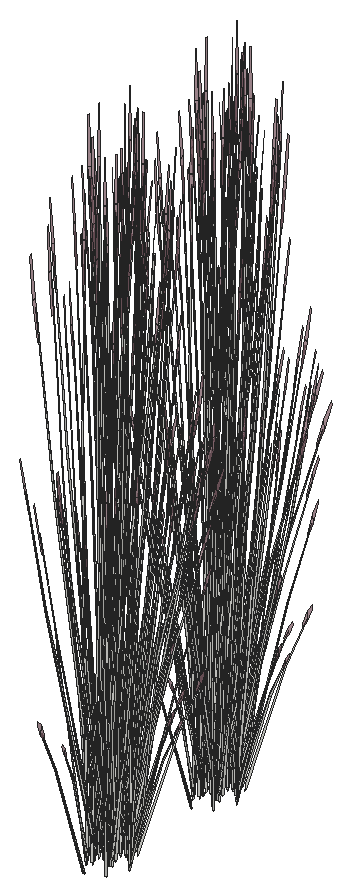
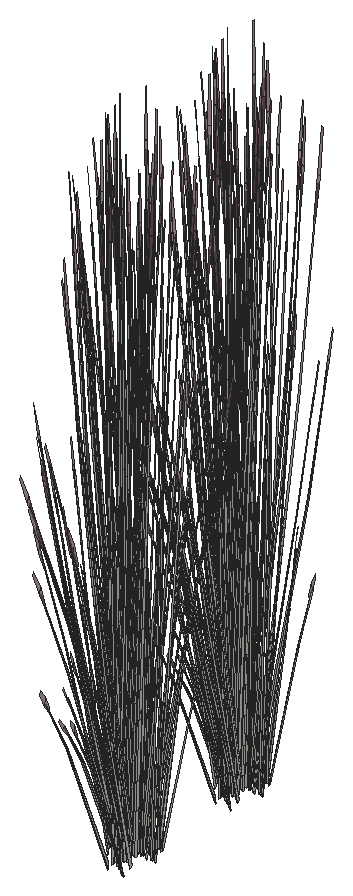
# SketchUp Ruby script. Lengths in inches.
U = 1.inch
M = Sketchup.active_model
def pt(a) = Geom::Point3d.new(a.map { |v| v * U })
def face(e, loops, mat)
  f = e.add_face(loops[0].map { |a| pt(a) })
  loops[1..].each { |l| e.add_face(l.map { |a| pt(a) }).erase! }
  f.material = f.back_material = mat if mat
  f
end
# faces: each face lists its corners as indices into pts; further lists are holes
def faces(e, pts, list, mat = nil) = list.each { |f| face(e, (f[0].is_a?(Array) ? f : [f]).map { |l| l.map { |i| pts[i] } }, mat) }
# xy, xz, yz: faces in a plane at the given z, y or x. An outline is a flat list of corners, or four numbers for a rectangle; further outlines are holes
def ring(l) = l.size == 4 ? [[l[0], l[1]], [l[2], l[1]], [l[2], l[3]], [l[0], l[3]]] : l.each_slice(2).to_a
def flat(e, list, mat, &to3) = list.each { |f| face(e, (f[0].is_a?(Array) ? f : [f]).map { |l| ring(l).map { |u, v| to3.(u, v) } }, mat) }
def xy(e, z, list, mat = nil) = flat(e, list, mat) { |x, y| [x, y, z] }
def xz(e, y, list, mat = nil) = flat(e, list, mat) { |x, z| [x, y, z] }
def yz(e, x, list, mat = nil) = flat(e, list, mat) { |y, z| [x, y, z] }
def lines(e, pts, list) = list.each { |a, b| e.add_line(pt(pts[a]), pt(pts[b])) }
# prism: a flat outline (further loops are holes) pulled along v
def prism(e, loops, v, mat = nil)
  f = face(e, loops, mat); d = Geom::Vector3d.new(v.map { |x| x * U })
  f.pushpull(f.normal.samedirection?(d) ? d.length : -d.length)
end
def box(e, o, s, mat = nil) = prism(e, [[o, [o[0] + s[0], o[1], o[2]], [o[0] + s[0], o[1] + s[1], o[2]], [o[0], o[1] + s[1], o[2]]]], [0, 0, s[2]], mat)
def at(x, y, z, deg = 0) = Geom::Transformation.translation(pt([x, y, z])) * Geom::Transformation.rotation(ORIGIN, Z_AXIS, deg.degrees)
def axes(o, x, y, z) = Geom::Transformation.new([*x, 0, *y, 0, *z, 0, *pt(o).to_a, 1])
def part(name) = M.definitions.add(name)
# library, detail: a bought-in or finely detailed component or shape, given as its bounding box
def library(name, o, s) = part(name).tap { |d| box(d.entities, o, s) }
def detail(e, o, s) = box(e.add_group.entities, o, s)
def put(e, d, t, mat = nil) = e.add_instance(d, t).tap { |i| i.material = mat if mat }
def group(e, t, mat = nil) = e.add_group.tap { |g| g.transformation = t; g.material = mat if mat }.entities
root = M.entities
M.materials.add("LightPink_Translucent").color = [144, 107, 117]
M.materials["LightPink_Translucent"].alpha = 0.75
c1 = part("blade")
p = [[2.15,0.21,22],[0,0.17,0],[0.09,0.45,0],[2.18,0.31,22],[2.29,0.31,22],[0.38,0.45,0],
  [2.48,0.24,33],[2.49,0.24,33],[2.48,0.22,33]]
faces(c1.entities,p,[[0,1,2,3],[4,5,2,3],[6,3,4,7],[8,0,3,6]])
c2 = part("seeds")
p = [[0.3,-0.1,1.38],[-0.01,-0.03,1.59],[-0.01,-0.03,0.03],[0.14,-0.07,-0.07],[0.29,-0.03,3],[0.15,0.01,3.11]]
faces(c2.entities,p,[[0,1,2,3],[1,0,4,5]],"LightPink_Translucent")
c3 = part("blade with seeds")
put(c3.entities,c1,at(0,0,0))
put(c3.entities,c2,axes([2.4,0.25,30.99],[1.5799,-0.05474,1.17369],[-0.12525,1.92788,0.29478],[-0.07173,-0.02425,1.56792]))
put(root,c3,axes([401.98,775.3,1.49],[-0.0592,0.0168,1.76342],[-0.32738,-0.18913,-0.26939],[0.00549,-0.15776,0.30037]))
put(root,c3,axes([402.97,776.51,4.98],[0.00918,-0.43138,-0.71045],[0.38672,0.02897,0.08574],[0.04081,-0.18275,1.00501]))
put(root,c3,axes([402.3,775.82,4.53],[0.1064,-0.35863,-0.35414],[0.31043,0.1046,0.4572],[-0.02846,-0.14439,0.87481]))
put(root,c3,axes([402.53,776.3,3.875],[-0.06572,0.16029,1.71376],[-0.27569,-0.33172,0.13857],[0.12437,-0.20675,0.73262]))
put(root,c3,axes([402.14,776.07,4.68],[-0.34695,-0.11691,-0.51099],[0.11892,-0.40083,-0.3958],[-0.03181,-0.16138,0.97773]))
put(root,c3,axes([402.35,775.0625,2.77],[0.04528,0.27194,1.1486],[-0.25117,-0.15062,0.84392],[0.02703,-0.13924,0.25299]))
put(root,c3,axes([402.89,776.37,4.68],[-0.25266,-0.31335,-0.51099],[0.2669,-0.27442,-0.3958],[0.03844,-0.15921,0.97773]))
put(root,c3,axes([403.13,776.26,4.53],[0.23881,-0.24554,-0.35414],[0.22606,0.28036,0.4572],[0.0344,-0.14245,0.87481]))
put(root,c3,axes([401.49,777.57,2.1],[-0.14494,-0.47823,-0.69835],[0.41752,-0.17223,-0.18329],[-0.01602,-0.16194,1.54149]))
put(root,c3,axes([403.43,776.11,1.49],[-0.05283,-0.03674,1.76342],[-0.13569,-0.41045,-0.26939],[0.09154,-0.11138,0.30037]))
put(root,c3,axes([403.42,777.26,4.98],[0.18436,-0.36797,-0.71045],[0.32306,0.26151,0.08574],[0.11008,-0.13332,1.00501]))
put(root,c3,axes([401.43,776.19,2.375],[-0.22066,-0.46731,0],[0.36918,-0.26061,-0.51607],[0.08408,-0.05936,1.63711]))
put(root,c3,axes([403.41,777.09,4.68],[-0.09067,-0.42583,-0.51099],[0.34336,-0.07449,-0.3958],[0.0984,-0.11438,0.97773]))
put(root,c3,axes([401.92,775.63,2.13],[-0.2439,0.26754,-0.03893],[-0.22348,-0.29302,-0.17649],[-0.01573,-0.08303,0.58215]))
put(root,c3,axes([400.63,777.5,2.02],[0,-0.46636,-0.49651],[0.39487,0,0],[0,-0.10622,1.57504]))
put(root,c3,axes([401.73,776.12,2.02],[0.33032,-0.23318,-0.49651],[0.19744,0.41812,0],[0.07523,-0.05311,1.57504]))
put(root,c3,axes([403.69,776.93,2.59],[-0.12609,-0.01381,1.43002],[-0.12917,-0.37055,-0.30754],[0.1549,-0.10482,0.61141]))
put(root,c3,axes([402.12,777.08,2.06],[0.23773,-0.35053,-0.62353],[0.29532,0.31785,-0.16365],[0.09526,-0.08744,1.37633]))
put(root,c3,axes([403.84,776.25,2.77],[-0.11756,0.2374,1.1486],[-0.10105,-0.31895,0.84392],[0.09709,-0.07992,0.25299]))
put(root,c3,axes([403.67,777.14,4.53],[0.30722,-0.06665,-0.35414],[0.08112,0.381,0.4572],[0.08804,-0.10234,0.87481]))
put(root,c3,axes([401.71,777.69,2.21],[0.17124,-0.42022,-0.44739],[0.35581,0.20224,0.21531],[0,-0.09687,1.43643]))
put(root,c3,axes([401.86,777.48,2.67],[-0.04113,-0.53214,-0.29095],[0.42835,-0.03218,-0.50002],[0.07543,-0.07088,1.59708]))
put(root,c3,axes([400.8,777.51,2.03],[0.24637,-0.29097,-0.30978],[0.24637,0.29097,0.30978],[0,-0.09372,1.38974]))
put(root,c3,axes([401.67,778.04,2.67],[-0.39748,-0.22252,-0.29095],[0.19139,-0.46966,-0.50002],[-0.01249,-0.11531,1.59708]))
put(root,c3,axes([401.81,776.31,2.03],[0.32928,0.11539,-0.30978],[-0.08291,0.40636,0.30978],[0.06638,-0.04686,1.38974]))
put(root,c3,axes([401.92,777.9,2.43],[0.39767,0.22603,0.24065],[-0.19139,0.46966,0.50002],[0,-0.10827,1.60543]))
put(root,c3,axes([401.79,777.59,2.72],[-0.38326,0.02879,0.44739],[-0.03466,-0.47788,-0.21531],[0.06861,-0.04843,1.43643]))
put(root,c3,axes([400.8,777.93,2.48],[0,0.46636,0.49651],[-0.39487,0,0],[0,-0.10622,1.57504]))
put(root,c3,axes([403.57,778.04,4.68],[0.09562,-0.42421,-0.51099],[0.32782,0.1454,-0.3958],[0.13199,-0.0389,0.97773]))
put(root,c3,axes([403.06,776.3125,2.375],[0.22066,-0.46731,0],[0.36918,0.26061,-0.51607],[0.08408,0.05936,1.63711]))
put(root,c3,axes([401.78,777.76,2.36],[0.15345,0.52148,0.45755],[-0.43845,0.18134,0.17955],[0.00536,-0.09582,1.58856]))
put(root,c3,axes([403.92,778.16,1.98],[-0.22732,0.05597,1.41583],[-0.03618,-0.44548,0.08104],[0.15921,-0.06743,0.80566]))
put(root,c3,axes([404.34,777.76,2.26],[-0.21881,-0.29821,-0.06488],[0.23965,-0.27324,-0.29416],[0.0679,-0.01924,0.97024]))
put(root,c3,axes([401.7,778.17,2.72],[-0.17124,0.42022,0.44739],[-0.35581,-0.20224,-0.21531],[0,-0.09687,1.43643]))
put(root,c3,axes([402.33,777.8,2.21],[0,-0.53961,0],[0.44133,0,0],[0,0,1.79456]))
put(root,c3,axes([402.87,776.56,2.48],[-0.33032,-0.23318,0.49651],[0.19744,-0.41812,0],[0.07523,0.05311,1.57504]))
put(root,c3,axes([403.51,778.19,4.98],[0.31014,-0.20596,-0.71045],[0.17284,0.42397,0.08574],[0.14985,-0.04816,1.00501]))
put(root,c3,axes([402.12,777.46,2.36],[-0.29264,0.42323,0.45755],[-0.34767,-0.3736,0.17955],[0.07055,-0.04224,1.58856]))
put(root,c3,axes([402.44,778.22,2.3],[-0.32829,-0.4014,-0.06131],[0.32849,-0.40164,0],[-0.01146,-0.01402,1.75571]))
put(root,c3,axes([401.61,776.77,2.47],[-0.10196,0.46348,0.17642],[-0.3731,-0.13116,0.35086],[0.06445,-0.00226,1.60407]))
put(root,c3,axes([401.46,777.14,1.59],[-0.3474,0.18671,1.28929],[-0.11057,-0.53572,0.50096],[0.21332,0.00891,1.46642]))
put(root,c3,axes([402.39,777.28,2.62],[0.06809,-0.4162,0.1448],[0.33266,0.07225,-0.41347],[0.06054,0.04274,1.26744]))
put(root,c3,axes([401.82,778.27,2.36],[0.44609,0.09826,0.45755],[-0.09078,0.55493,0.17955],[-0.06519,-0.05359,1.58856]))
put(root,c3,axes([404.17,777.87,1.49],[-0.01845,-0.0708,1.76342],[0.12793,-0.41416,-0.26939],[0.12905,-0.00596,0.30037]))
put(root,c3,axes([402.25,777.39,2.72],[-0.21202,-0.39143,0.44739],[0.32115,-0.27564,-0.21531],[0.06861,0.04843,1.43643]))
put(root,c3,axes([401.58,779.16,2.47],[0.37926,-0.12378,0.17642],[0.09365,0.46065,0.35086],[-0.03382,-0.06712,1.60407]))
put(root,c3,axes([402.36,777.42,2.67],[0.35635,-0.30962,-0.29095],[0.23697,0.43749,-0.50002],[0.08792,0.04443,1.59708]))
put(root,c3,axes([403.78,778.23,4.53],[0.29332,0.1301,-0.35414],[-0.08555,0.37955,0.4572],[0.11809,-0.0348,0.87481]))
put(root,c3,axes([403.26,776.59,2.02],[0.33032,0.23318,-0.49651],[-0.19744,0.41812,0],[0.07523,0.05311,1.57504]))
put(root,c3,axes([402.63,777.92,2.21],[0.39487,0,0],[0,0.48281,0],[0,0,1.78407]))
put(root,c3,axes([402.74,776.79,2.47],[-0.37926,0.12378,0.17642],[-0.09365,-0.46065,0.35086],[0.03382,0.06712,1.60407]))
put(root,c3,axes([402.98,777.76,3.875],[-0.14639,0.01056,1.71376],[0.09712,-0.45778,0.13857],[0.20862,0.02831,0.73262]))
put(root,c3,axes([403.17,776.77,2.03],[0.08291,0.40636,-0.30978],[-0.32928,0.11539,0.30978],[0.06638,0.04686,1.38974]))
put(root,c3,axes([402.5,777.68,2.38],[-0.44609,-0.09826,0.49198],[0.09078,-0.55493,0.19306],[0.06519,0.05359,1.70813]))
put(root,c3,axes([402.15,779.05,2.2],[-0.11516,-0.40207,0],[0.32884,-0.1408,0],[0,0,1.54371]))
put(root,c3,axes([402.58,778.99,2.18],[0.37054,-0.15823,-0.19198],[0.1302,0.45581,0.00008],[0.0409,-0.01749,1.73897]))
put(root,c3,axes([402.71,779.18,2.47],[0.10196,-0.46348,0.17642],[0.3731,0.13116,0.35086],[-0.06445,0.00226,1.60407]))
put(root,c3,axes([402.62,778.13,2.21],[0.24637,0.30123,0],[-0.24637,0.30123,0],[0,0,1.69266]))
put(root,c3,axes([403.29,778,2.47],[-0.2773,-0.3397,0.17642],[0.27945,-0.32949,0.35086],[-0.03063,0.06937,1.60407]))
put(root,c3,axes([402.78,777.49,2.06],[0.36714,0.07646,-0.62353],[-0.07747,0.47163,-0.16365],[0.10956,0.05715,1.37633]))
put(root,c3,axes([404.4,778.31,2.77],[-0.21807,0.07699,1.1486],[0.10265,-0.31819,0.84392],[0.11568,0.02177,0.25299]))
put(root,c3,axes([402.07,779.23,2.2],[-0.35581,-0.20937,0],[0.17124,-0.43505,0],[0,0,1.62707]))
put(root,c3,axes([402.62,777.78,2.72],[0.17124,-0.42022,0.44739],[0.35581,0.20224,-0.21531],[0,0.09687,1.43643]))
put(root,c3,axes([402.55,778.02,2.29],[0,0.53934,-0.05637],[-0.44133,0,0],[0,0.01695,1.79368]))
put(root,c3,axes([402.58,777.64,2.21],[0.21202,0.39143,-0.44739],[-0.32115,0.27564,0.21531],[0.06861,0.04843,1.43643]))
put(root,c3,axes([404.02,779.29,3.93],[-0.06755,-0.39203,-0.03492],[0.31928,-0.09013,-0.15832],[0.06667,0.02485,0.52218]))
put(root,c3,axes([403.52,778.01,2.48],[0,-0.46636,0.49651],[0.39487,0,0],[0,0.10622,1.57504]))
put(root,c3,axes([402.53,778.36,2.72],[0.38326,-0.02879,0.44739],[0.03466,0.47788,-0.21531],[-0.06861,0.04843,1.43643]))
put(root,c3,axes([402.77,777.875,2.62],[0.32884,-0.136,0.1448],[0.11516,0.38837,-0.41347],[0,0.08547,1.26744]))
put(root,c3,axes([403.99,778.82,2.59],[-0.085,-0.1147,1.43002],[0.1106,-0.37943,-0.30754],[0.17198,0.0514,0.61141]))
put(root,c3,axes([402.47,779.24,2.2],[0.35581,0.20937,0],[-0.17124,0.43505,0],[0,0,1.74954]))
put(root,c3,axes([402.61,779.7,2.19],[-0.21791,-0.46895,-0.05142],[0.36918,-0.26061,0.51607],[-0.09097,0.04465,1.6363]))
put(root,c3,axes([402.53,778.57,2.62],[0.26075,0.2802,0.1448],[-0.2175,0.31612,-0.41347],[-0.06054,0.04274,1.26744]))
put(root,c3,axes([403.21,779.05,4.98],[0.35281,0.01123,-0.71045],[-0.0237,0.47284,0.08574],[0.14947,0.0499,1.00501]))
put(root,c3,axes([402.8125,779.43,2.48],[0.33032,-0.23318,0.49651],[0.19744,0.41812,0],[-0.07523,0.05311,1.57504]))
put(root,c3,axes([402.34,779.0625,2.29],[0.15345,0.53576,-0.06012],[-0.43845,0.18773,0],[0.00536,0.01871,1.72173]))
put(root,c3,axes([402.51,779.64,2.03],[-0.32928,-0.11539,-0.30978],[0.08291,-0.40636,0.30978],[-0.06638,0.04686,1.38974]))
put(root,c3,axes([403.78,778.09,2.375],[0.44133,0,0],[0,0.52122,-0.51607],[0,0.11871,1.63711]))
put(root,c3,axes([403.61,778.36,2.2],[-0.44111,-0.00373,-0.04976],[0,-0.52122,0.49943],[-0.01386,0.11865,1.58352]))
put(root,c3,axes([402.65,777.9,2.67],[0.39748,0.22252,-0.29095],[-0.19139,0.46966,-0.50002],[0.01249,0.11531,1.59708]))
put(root,c3,axes([403.42,779.25,4.53],[0.20082,0.29199,-0.35414],[-0.2293,0.2764,0.4572],[0.1165,0.04206,0.87481]))
put(root,c3,axes([403.52,778.43,2.03],[-0.24637,0.29097,-0.30978],[-0.24637,-0.29097,0.30978],[0,0.09372,1.38974]))
put(root,c3,axes([402.46,778.46,2.67],[0.04113,0.53214,-0.29095],[-0.42835,0.03218,-0.50002],[-0.07543,0.07088,1.59708]))
put(root,c3,axes([402.61,778.25,2.21],[-0.17124,0.42022,-0.44739],[-0.35581,-0.20224,0.21531],[0,0.09687,1.43643]))
put(root,c3,axes([402.62,779.46,2.33],[0.44186,0.15158,0.30756],[-0.11054,0.54181,-0.36492],[-0.07313,0.06781,1.64885]))
put(root,c3,axes([402.59,779.82,2.02],[-0.33032,0.23318,-0.49651],[-0.19744,-0.41812,0],[-0.07523,0.05311,1.57504]))
put(root,c3,axes([403.6875,778.44,2.02],[0,0.46636,-0.49651],[-0.39487,0,0],[0,0.10622,1.57504]))
put(root,c3,axes([402.7,778.5,3.875],[-0.1311,-0.08035,1.71376],[0.27131,-0.33708,0.13857],[0.16909,0.15206,0.73262]))
put(root,c3,axes([403.18,779.41,2.77],[-0.19872,-0.13409,1.1486],[0.2566,-0.13625,0.84392],[0.06921,0.11541,0.25299]))
put(root,c3,axes([402.89,779.75,2.375],[0.22066,0.46731,0],[-0.36918,0.26061,-0.51607],[-0.08408,0.05936,1.63711]))
put(root,c3,axes([403.24,779.91,1.49],[0.02571,-0.06733,1.76342],[0.32373,-0.19829,-0.26939],[0.09815,0.10263,0.30037]))
put(root,c3,axes([402.7,777.9,2.84],[-0.00964,-0.43909,1.41272],[0.43635,0.11382,0.59816],[-0.1032,0.24027,1.3335]))
put(root,c3,axes([402.8125,778.38,2.09],[0.12941,0.42699,-0.69212],[-0.37279,0.15378,-0.18165],[0.0143,0.14459,1.52773]))
put(root,c3,axes([402.74,779.6,4.68],[0.34827,-0.11086,-0.51099],[0.06092,0.41983,-0.3958],[0.09354,0.12031,0.97773]))
put(root,c3,axes([403.22,780.02,2.67],[-0.22633,-0.01463,1.0506],[0.14947,-0.31064,0.58006],[0.08941,0.11036,0.8241]))
put(root,c3,axes([402.48,779.27,2.59],[0.00623,-0.15459,1.43002],[0.29764,-0.17268,-0.30754],[0.09188,0.18503,0.61141]))
put(root,c3,axes([401.73,779.89,1.49],[0.05712,-0.02538,1.76342],[0.34359,0.13968,-0.26939],[0.01005,0.15742,0.30037]))
put(root,c3,axes([401.21,779.49,5],[0.25266,0.31335,-0.5672],[-0.2669,0.27442,-0.43934],[-0.03844,0.15921,1.08528]))
put(root,c3,axes([400.9375,779.96,2.82],[0.32063,-0.08258,0.06507],[0.07371,0.33271,-0.86304],[-0.02033,0.16842,0.7736]))
put(root,c3,axes([401.96,779.79,4.68],[0.34695,0.11691,-0.51099],[-0.11892,0.40083,-0.3958],[0.03181,0.16138,0.97773]))
put(root,c3,axes([402.16,778.96,3.875],[-0.08068,-0.14973,1.71376],[0.3728,-0.12606,0.13857],[0.08426,0.23506,0.73262]))
put(root,c3,axes([401.8,780.04,4.53],[-0.1064,0.35863,-0.35414],[-0.31043,-0.1046,0.4572],[0.02846,0.14439,0.87481]))
put(root,c3,axes([401.5,779.04,3.875],[-0.00864,-0.17899,1.71376],[0.37441,0.11874,0.13857],[-0.02316,0.25508,0.73262]))
put(root,c3,axes([401.84,779.72,4.98],[0.16845,0.3792,-0.71045],[-0.34676,0.21133,0.08574],[0.03939,0.18322,1.00501]))
put(root,c3,axes([402.72,788.58,2.59],[-0.10032,0.0944,1.43002],[-0.30046,-0.16522,-0.30754],[0.05569,-0.20547,0.61141]))
put(root,c3,axes([402.27,788.91,4.98],[-0.16845,-0.3792,-0.71045],[0.34676,-0.21133,0.08574],[-0.03939,-0.18322,1.00501]))
put(root,c3,axes([401.98,788.07,1.49],[-0.0592,0.0168,1.76342],[-0.32738,-0.18913,-0.26939],[0.00549,-0.15776,0.30037]))
put(root,c3,axes([402.97,789.28,4.98],[0.00918,-0.43138,-0.71045],[0.38672,0.02897,0.08574],[0.04081,-0.18275,1.00501]))
put(root,c3,axes([402.3,788.59,4.53],[0.1064,-0.35863,-0.35414],[0.31043,0.1046,0.4572],[-0.02846,-0.14439,0.87481]))
put(root,c3,axes([402.53,789.06,3.875],[-0.06572,0.16029,1.71376],[-0.27569,-0.33172,0.13857],[0.12437,-0.20675,0.73262]))
put(root,c3,axes([402.14,788.84,4.68],[-0.34695,-0.11691,-0.51099],[0.11892,-0.40083,-0.3958],[-0.03181,-0.16138,0.97773]))
put(root,c3,axes([402.35,787.83,2.77],[0.04528,0.27194,1.1486],[-0.25117,-0.15062,0.84392],[0.02703,-0.13924,0.25299]))
put(root,c3,axes([402.89,789.14,4.68],[-0.25266,-0.31335,-0.51099],[0.2669,-0.27442,-0.3958],[0.03844,-0.15921,0.97773]))
put(root,c3,axes([403.13,789.02,4.53],[0.23881,-0.24554,-0.35414],[0.22606,0.28036,0.4572],[0.0344,-0.14245,0.87481]))
put(root,c3,axes([401.49,790.34,2.1],[-0.14494,-0.47823,-0.69835],[0.41752,-0.17223,-0.18329],[-0.01602,-0.16194,1.54149]))
put(root,c3,axes([403.43,788.875,1.49],[-0.05283,-0.03674,1.76342],[-0.13569,-0.41045,-0.26939],[0.09154,-0.11138,0.30037]))
put(root,c3,axes([403.42,790.03,4.98],[0.18436,-0.36797,-0.71045],[0.32306,0.26151,0.08574],[0.11008,-0.13332,1.00501]))
put(root,c3,axes([401.43,788.96,2.375],[-0.22066,-0.46731,0],[0.36918,-0.26061,-0.51607],[0.08408,-0.05936,1.63711]))
put(root,c3,axes([403.41,789.86,4.68],[-0.09067,-0.42583,-0.51099],[0.34336,-0.07449,-0.3958],[0.0984,-0.11438,0.97773]))
put(root,c3,axes([401.92,788.4,2.13],[-0.2439,0.26754,-0.03893],[-0.22348,-0.29302,-0.17649],[-0.01573,-0.08303,0.58215]))
put(root,c3,axes([400.63,790.27,2.02],[0,-0.46636,-0.49651],[0.39487,0,0],[0,-0.10622,1.57504]))
put(root,c3,axes([401.73,788.89,2.02],[0.33032,-0.23318,-0.49651],[0.19744,0.41812,0],[0.07523,-0.05311,1.57504]))
put(root,c3,axes([403.69,789.7,2.59],[-0.12609,-0.01381,1.43002],[-0.12917,-0.37055,-0.30754],[0.1549,-0.10482,0.61141]))
put(root,c3,axes([402.12,789.85,2.06],[0.23773,-0.35053,-0.62353],[0.29532,0.31785,-0.16365],[0.09526,-0.08744,1.37633]))
put(root,c3,axes([403.84,789.01,2.77],[-0.11756,0.2374,1.1486],[-0.10105,-0.31895,0.84392],[0.09709,-0.07992,0.25299]))
put(root,c3,axes([403.67,789.91,4.53],[0.30722,-0.06665,-0.35414],[0.08112,0.381,0.4572],[0.08804,-0.10234,0.87481]))
put(root,c3,axes([401.71,790.46,2.21],[0.17124,-0.42022,-0.44739],[0.35581,0.20224,0.21531],[0,-0.09687,1.43643]))
put(root,c3,axes([401.86,790.25,2.67],[-0.04113,-0.53214,-0.29095],[0.42835,-0.03218,-0.50002],[0.07543,-0.07088,1.59708]))
put(root,c3,axes([400.8,790.28,2.03],[0.24637,-0.29097,-0.30978],[0.24637,0.29097,0.30978],[0,-0.09372,1.38974]))
put(root,c3,axes([401.67,790.81,2.67],[-0.39748,-0.22252,-0.29095],[0.19139,-0.46966,-0.50002],[-0.01249,-0.11531,1.59708]))
put(root,c3,axes([401.81,789.07,2.03],[0.32928,0.11539,-0.30978],[-0.08291,0.40636,0.30978],[0.06638,-0.04686,1.38974]))
put(root,c3,axes([401.92,790.67,2.43],[0.39767,0.22603,0.24065],[-0.19139,0.46966,0.50002],[0,-0.10827,1.60543]))
put(root,c3,axes([401.79,790.35,2.72],[-0.38326,0.02879,0.44739],[-0.03466,-0.47788,-0.21531],[0.06861,-0.04843,1.43643]))
put(root,c3,axes([400.8,790.7,2.48],[0,0.46636,0.49651],[-0.39487,0,0],[0,-0.10622,1.57504]))
put(root,c3,axes([403.57,790.81,4.68],[0.09562,-0.42421,-0.51099],[0.32782,0.1454,-0.3958],[0.13199,-0.0389,0.97773]))
put(root,c3,axes([403.06,789.08,2.375],[0.22066,-0.46731,0],[0.36918,0.26061,-0.51607],[0.08408,0.05936,1.63711]))
put(root,c3,axes([401.78,790.53,2.36],[0.15345,0.52148,0.45755],[-0.43845,0.18134,0.17955],[0.00536,-0.09582,1.58856]))
put(root,c3,axes([403.92,790.93,1.98],[-0.22732,0.05597,1.41583],[-0.03618,-0.44548,0.08104],[0.15921,-0.06743,0.80566]))
put(root,c3,axes([404.34,790.53,2.26],[-0.21881,-0.29821,-0.06488],[0.23965,-0.27324,-0.29416],[0.0679,-0.01924,0.97024]))
put(root,c3,axes([401.7,790.9375,2.72],[-0.17124,0.42022,0.44739],[-0.35581,-0.20224,-0.21531],[0,-0.09687,1.43643]))
put(root,c3,axes([402.33,790.57,2.21],[0,-0.53961,0],[0.44133,0,0],[0,0,1.79456]))
put(root,c3,axes([402.87,789.32,2.48],[-0.33032,-0.23318,0.49651],[0.19744,-0.41812,0],[0.07523,0.05311,1.57504]))
put(root,c3,axes([403.51,790.96,4.98],[0.31014,-0.20596,-0.71045],[0.17284,0.42397,0.08574],[0.14985,-0.04816,1.00501]))
put(root,c3,axes([402.12,790.23,2.36],[-0.29264,0.42323,0.45755],[-0.34767,-0.3736,0.17955],[0.07055,-0.04224,1.58856]))
put(root,c3,axes([402.44,790.99,2.3],[-0.32829,-0.4014,-0.06131],[0.32849,-0.40164,0],[-0.01146,-0.01402,1.75571]))
put(root,c3,axes([401.61,789.53,2.47],[-0.10196,0.46348,0.17642],[-0.3731,-0.13116,0.35086],[0.06445,-0.00226,1.60407]))
put(root,c3,axes([401.46,789.91,1.59],[-0.3474,0.18671,1.28929],[-0.11057,-0.53572,0.50096],[0.21332,0.00891,1.46642]))
put(root,c3,axes([402.39,790.05,2.62],[0.06809,-0.4162,0.1448],[0.33266,0.07225,-0.41347],[0.06054,0.04274,1.26744]))
put(root,c3,axes([401.82,791.04,2.36],[0.44609,0.09826,0.45755],[-0.09078,0.55493,0.17955],[-0.06519,-0.05359,1.58856]))
put(root,c3,axes([404.17,790.64,1.49],[-0.01845,-0.0708,1.76342],[0.12793,-0.41416,-0.26939],[0.12905,-0.00596,0.30037]))
put(root,c3,axes([402.25,790.16,2.72],[-0.21202,-0.39143,0.44739],[0.32115,-0.27564,-0.21531],[0.06861,0.04843,1.43643]))
put(root,c3,axes([401.58,791.92,2.47],[0.37926,-0.12378,0.17642],[0.09365,0.46065,0.35086],[-0.03382,-0.06712,1.60407]))
put(root,c3,axes([402.36,790.18,2.67],[0.35635,-0.30962,-0.29095],[0.23697,0.43749,-0.50002],[0.08792,0.04443,1.59708]))
put(root,c3,axes([403.78,791,4.53],[0.29332,0.1301,-0.35414],[-0.08555,0.37955,0.4572],[0.11809,-0.0348,0.87481]))
put(root,c3,axes([403.26,789.36,2.02],[0.33032,0.23318,-0.49651],[-0.19744,0.41812,0],[0.07523,0.05311,1.57504]))
put(root,c3,axes([402.63,790.69,2.21],[0.39487,0,0],[0,0.48281,0],[0,0,1.78407]))
put(root,c3,axes([402.74,789.56,2.47],[-0.37926,0.12378,0.17642],[-0.09365,-0.46065,0.35086],[0.03382,0.06712,1.60407]))
put(root,c3,axes([402.98,790.53,3.875],[-0.14639,0.01056,1.71376],[0.09712,-0.45778,0.13857],[0.20862,0.02831,0.73262]))
put(root,c3,axes([403.17,789.54,2.03],[0.08291,0.40636,-0.30978],[-0.32928,0.11539,0.30978],[0.06638,0.04686,1.38974]))
put(root,c3,axes([402.5,790.45,2.38],[-0.44609,-0.09826,0.49198],[0.09078,-0.55493,0.19306],[0.06519,0.05359,1.70813]))
put(root,c3,axes([402.15,791.82,2.2],[-0.11516,-0.40207,0],[0.32884,-0.1408,0],[0,0,1.54371]))
put(root,c3,axes([402.58,791.76,2.18],[0.37054,-0.15823,-0.19198],[0.1302,0.45581,0.00008],[0.0409,-0.01749,1.73897]))
put(root,c3,axes([402.71,791.95,2.47],[0.10196,-0.46348,0.17642],[0.3731,0.13116,0.35086],[-0.06445,0.00226,1.60407]))
put(root,c3,axes([402.62,790.9,2.21],[0.24637,0.30123,0],[-0.24637,0.30123,0],[0,0,1.69266]))
put(root,c3,axes([403.29,790.77,2.47],[-0.2773,-0.3397,0.17642],[0.27945,-0.32949,0.35086],[-0.03063,0.06937,1.60407]))
put(root,c3,axes([402.78,790.25,2.06],[0.36714,0.07646,-0.62353],[-0.07747,0.47163,-0.16365],[0.10956,0.05715,1.37633]))
put(root,c3,axes([404.4,791.08,2.77],[-0.21807,0.07699,1.1486],[0.10265,-0.31819,0.84392],[0.11568,0.02177,0.25299]))
put(root,c3,axes([402.07,792,2.2],[-0.35581,-0.20937,0],[0.17124,-0.43505,0],[0,0,1.62707]))
put(root,c3,axes([402.62,790.55,2.72],[0.17124,-0.42022,0.44739],[0.35581,0.20224,-0.21531],[0,0.09687,1.43643]))
put(root,c3,axes([402.55,790.79,2.29],[0,0.53934,-0.05637],[-0.44133,0,0],[0,0.01695,1.79368]))
put(root,c3,axes([402.58,790.4,2.21],[0.21202,0.39143,-0.44739],[-0.32115,0.27564,0.21531],[0.06861,0.04843,1.43643]))
put(root,c3,axes([404.02,792.06,3.93],[-0.06755,-0.39203,-0.03492],[0.31928,-0.09013,-0.15832],[0.06667,0.02485,0.52218]))
put(root,c3,axes([403.52,790.78,2.48],[0,-0.46636,0.49651],[0.39487,0,0],[0,0.10622,1.57504]))
put(root,c3,axes([402.53,791.13,2.72],[0.38326,-0.02879,0.44739],[0.03466,0.47788,-0.21531],[-0.06861,0.04843,1.43643]))
put(root,c3,axes([402.77,790.64,2.62],[0.32884,-0.136,0.1448],[0.11516,0.38837,-0.41347],[0,0.08547,1.26744]))
put(root,c3,axes([403.99,791.59,2.59],[-0.085,-0.1147,1.43002],[0.1106,-0.37943,-0.30754],[0.17198,0.0514,0.61141]))
put(root,c3,axes([402.47,792.01,2.2],[0.35581,0.20937,0],[-0.17124,0.43505,0],[0,0,1.74954]))
put(root,c3,axes([402.61,792.47,2.19],[-0.21791,-0.46895,-0.05142],[0.36918,-0.26061,0.51607],[-0.09097,0.04465,1.6363]))
put(root,c3,axes([402.53,791.33,2.62],[0.26075,0.2802,0.1448],[-0.2175,0.31612,-0.41347],[-0.06054,0.04274,1.26744]))
put(root,c3,axes([403.21,791.82,4.98],[0.35281,0.01123,-0.71045],[-0.0237,0.47284,0.08574],[0.14947,0.0499,1.00501]))
put(root,c3,axes([402.8125,792.2,2.48],[0.33032,-0.23318,0.49651],[0.19744,0.41812,0],[-0.07523,0.05311,1.57504]))
put(root,c3,axes([402.34,791.83,2.29],[0.15345,0.53576,-0.06012],[-0.43845,0.18773,0],[0.00536,0.01871,1.72173]))
put(root,c3,axes([402.51,792.41,2.03],[-0.32928,-0.11539,-0.30978],[0.08291,-0.40636,0.30978],[-0.06638,0.04686,1.38974]))
put(root,c3,axes([403.78,790.86,2.375],[0.44133,0,0],[0,0.52122,-0.51607],[0,0.11871,1.63711]))
put(root,c3,axes([403.61,791.13,2.2],[-0.44111,-0.00373,-0.04976],[0,-0.52122,0.49943],[-0.01386,0.11865,1.58352]))
put(root,c3,axes([402.65,790.67,2.67],[0.39748,0.22252,-0.29095],[-0.19139,0.46966,-0.50002],[0.01249,0.11531,1.59708]))
put(root,c3,axes([403.42,792.01,4.53],[0.20082,0.29199,-0.35414],[-0.2293,0.2764,0.4572],[0.1165,0.04206,0.87481]))
put(root,c3,axes([403.52,791.2,2.03],[-0.24637,0.29097,-0.30978],[-0.24637,-0.29097,0.30978],[0,0.09372,1.38974]))
put(root,c3,axes([402.46,791.23,2.67],[0.04113,0.53214,-0.29095],[-0.42835,0.03218,-0.50002],[-0.07543,0.07088,1.59708]))
put(root,c3,axes([402.61,791.02,2.21],[-0.17124,0.42022,-0.44739],[-0.35581,-0.20224,0.21531],[0,0.09687,1.43643]))
put(root,c3,axes([402.62,792.23,2.33],[0.44186,0.15158,0.30756],[-0.11054,0.54181,-0.36492],[-0.07313,0.06781,1.64885]))
put(root,c3,axes([402.59,792.59,2.02],[-0.33032,0.23318,-0.49651],[-0.19744,-0.41812,0],[-0.07523,0.05311,1.57504]))
put(root,c3,axes([403.6875,791.21,2.02],[0,0.46636,-0.49651],[-0.39487,0,0],[0,0.10622,1.57504]))
put(root,c3,axes([402.7,791.27,3.875],[-0.1311,-0.08035,1.71376],[0.27131,-0.33708,0.13857],[0.16909,0.15206,0.73262]))
put(root,c3,axes([403.18,792.18,2.77],[-0.19872,-0.13409,1.1486],[0.2566,-0.13625,0.84392],[0.06921,0.11541,0.25299]))
put(root,c3,axes([402.89,792.52,2.375],[0.22066,0.46731,0],[-0.36918,0.26061,-0.51607],[-0.08408,0.05936,1.63711]))
put(root,c3,axes([403.24,792.68,1.49],[0.02571,-0.06733,1.76342],[0.32373,-0.19829,-0.26939],[0.09815,0.10263,0.30037]))
put(root,c3,axes([402.7,790.67,2.84],[-0.00964,-0.43909,1.41272],[0.43635,0.11382,0.59816],[-0.1032,0.24027,1.3335]))
put(root,c3,axes([402.8125,791.15,2.09],[0.12941,0.42699,-0.69212],[-0.37279,0.15378,-0.18165],[0.0143,0.14459,1.52773]))
put(root,c3,axes([402.74,792.37,4.68],[0.34827,-0.11086,-0.51099],[0.06092,0.41983,-0.3958],[0.09354,0.12031,0.97773]))
put(root,c3,axes([403.22,792.79,2.67],[-0.22633,-0.01463,1.0506],[0.14947,-0.31064,0.58006],[0.08941,0.11036,0.8241]))
put(root,c3,axes([402.48,792.04,2.59],[0.00623,-0.15459,1.43002],[0.29764,-0.17268,-0.30754],[0.09188,0.18503,0.61141]))
put(root,c3,axes([401.73,792.66,1.49],[0.05712,-0.02538,1.76342],[0.34359,0.13968,-0.26939],[0.01005,0.15742,0.30037]))
put(root,c3,axes([401.21,792.26,5],[0.25266,0.31335,-0.5672],[-0.2669,0.27442,-0.43934],[-0.03844,0.15921,1.08528]))
put(root,c3,axes([400.9375,792.73,2.82],[0.32063,-0.08258,0.06507],[0.07371,0.33271,-0.86304],[-0.02033,0.16842,0.7736]))
put(root,c3,axes([401.96,792.56,4.68],[0.34695,0.11691,-0.51099],[-0.11892,0.40083,-0.3958],[0.03181,0.16138,0.97773]))
put(root,c3,axes([402.16,791.73,3.875],[-0.08068,-0.14973,1.71376],[0.3728,-0.12606,0.13857],[0.08426,0.23506,0.73262]))
put(root,c3,axes([401.8,792.81,4.53],[-0.1064,0.35863,-0.35414],[-0.31043,-0.1046,0.4572],[0.02846,0.14439,0.87481]))
put(root,c3,axes([401.5,791.81,3.875],[-0.00864,-0.17899,1.71376],[0.37441,0.11874,0.13857],[-0.02316,0.25508,0.73262]))
put(root,c3,axes([401.84,792.48,4.98],[0.16845,0.3792,-0.71045],[-0.34676,0.21133,0.08574],[0.03939,0.18322,1.00501]))
